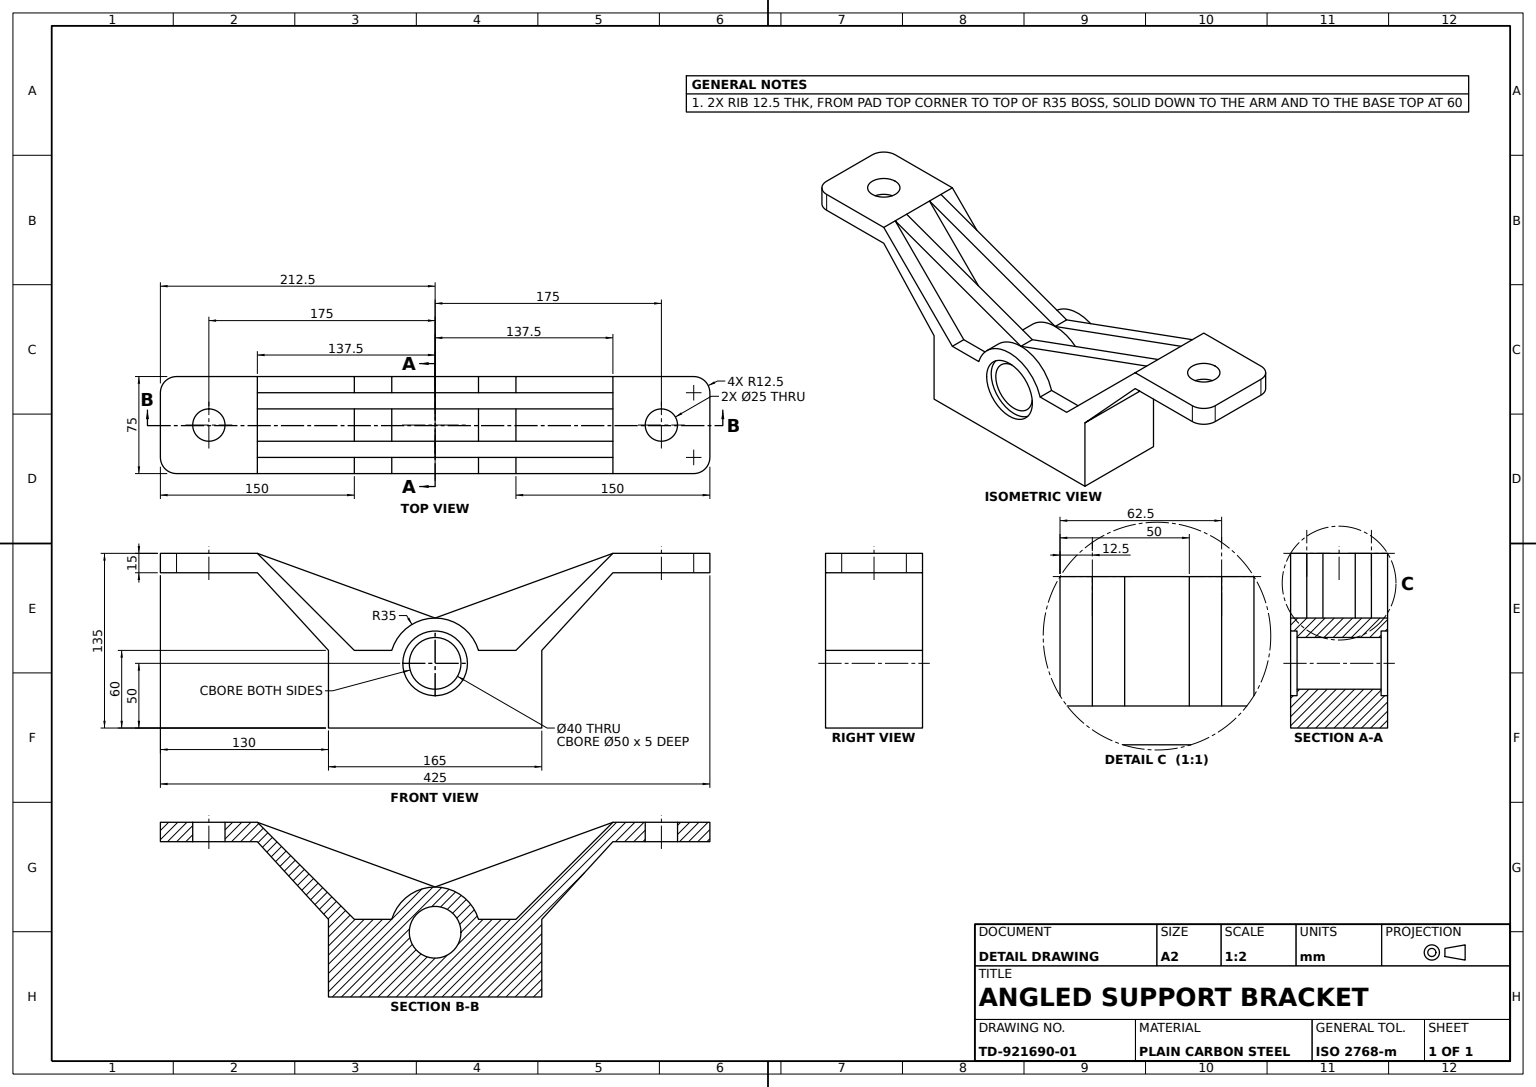
ISO-10303-21;
HEADER;
FILE_DESCRIPTION((''),'2;1');
FILE_NAME('','',(''),(''),'','','');
FILE_SCHEMA(('AUTOMOTIVE_DESIGN'));
ENDSEC;
DATA;
#1=APPLICATION_CONTEXT('');
#2=PRODUCT_CONTEXT('',#1,'mechanical');
#3=PRODUCT('','','',(#2));
#4=PRODUCT_DEFINITION_FORMATION('','',#3);
#5=PRODUCT_DEFINITION_CONTEXT('',#1,'design');
#6=PRODUCT_DEFINITION('','',#4,#5);
#7=PRODUCT_DEFINITION_SHAPE('','',#6);
#8=(LENGTH_UNIT()NAMED_UNIT(*)SI_UNIT(.MILLI.,.METRE.));
#9=(NAMED_UNIT(*)PLANE_ANGLE_UNIT()SI_UNIT($,.RADIAN.));
#10=(NAMED_UNIT(*)SI_UNIT($,.STERADIAN.)SOLID_ANGLE_UNIT());
#11=UNCERTAINTY_MEASURE_WITH_UNIT(LENGTH_MEASURE(1.E-05),#8,'distance_accuracy_value','');
#12=(GEOMETRIC_REPRESENTATION_CONTEXT(3)GLOBAL_UNCERTAINTY_ASSIGNED_CONTEXT((#11))GLOBAL_UNIT_ASSIGNED_CONTEXT((#8,#9,#10))REPRESENTATION_CONTEXT('',''));
#13=CARTESIAN_POINT('',(-212.5,90.,-62.5));
#14=VERTEX_POINT('',#13);
#15=CARTESIAN_POINT('',(-212.5,90.,-12.5));
#16=VERTEX_POINT('',#15);
#17=CARTESIAN_POINT('',(-212.5,90.,-75.));
#18=DIRECTION('',(0.,0.,1.));
#19=VECTOR('',#18,1000.);
#20=LINE('',#17,#19);
#21=EDGE_CURVE('',#14,#16,#20,.T.);
#22=ORIENTED_EDGE('',*,*,#21,.T.);
#23=CARTESIAN_POINT('',(-212.5,105.,-12.5));
#24=VERTEX_POINT('',#23);
#25=CARTESIAN_POINT('',(-212.5,0.,-12.5));
#26=DIRECTION('',(0.,1.,0.));
#27=VECTOR('',#26,1000.);
#28=LINE('',#25,#27);
#29=EDGE_CURVE('',#16,#24,#28,.T.);
#30=ORIENTED_EDGE('',*,*,#29,.T.);
#31=CARTESIAN_POINT('',(-212.5,105.,-62.5));
#32=VERTEX_POINT('',#31);
#33=CARTESIAN_POINT('',(-212.5,105.,-75.));
#34=LINE('',#33,#19);
#35=EDGE_CURVE('',#32,#24,#34,.T.);
#36=ORIENTED_EDGE('',*,*,#35,.F.);
#37=DIRECTION('',(0.,-1.,0.));
#38=VECTOR('',#37,1000.);
#39=LINE('',#13,#38);
#40=EDGE_CURVE('',#32,#14,#39,.T.);
#41=ORIENTED_EDGE('',*,*,#40,.T.);
#42=EDGE_LOOP('',(#22,#30,#36,#41));
#43=FACE_OUTER_BOUND('',#42,.T.);
#44=CARTESIAN_POINT('',(-212.5,0.,-75.));
#45=DIRECTION('',(-1.,0.,0.));
#46=AXIS2_PLACEMENT_3D('',#44,#45,#18);
#47=PLANE('',#46);
#48=ADVANCED_FACE('',(#43),#47,.T.);
#49=CARTESIAN_POINT('',(137.5,105.,-25.));
#50=VERTEX_POINT('',#49);
#51=CARTESIAN_POINT('',(62.5,30.,-25.));
#52=VERTEX_POINT('',#51);
#53=CARTESIAN_POINT('',(16.25,-16.25,-25.));
#54=DIRECTION('',(-0.707106781,-0.707106781,0.));
#55=VECTOR('',#54,1000.);
#56=LINE('',#53,#55);
#57=EDGE_CURVE('',#50,#52,#56,.T.);
#58=ORIENTED_EDGE('',*,*,#57,.F.);
#59=CARTESIAN_POINT('',(137.5,105.,-50.));
#60=VERTEX_POINT('',#59);
#61=CARTESIAN_POINT('',(137.5,105.,-75.));
#62=LINE('',#61,#19);
#63=EDGE_CURVE('',#60,#50,#62,.T.);
#64=ORIENTED_EDGE('',*,*,#63,.F.);
#65=CARTESIAN_POINT('',(62.5,30.,-50.));
#66=VERTEX_POINT('',#65);
#67=CARTESIAN_POINT('',(16.25,-16.25,-50.));
#68=LINE('',#67,#55);
#69=EDGE_CURVE('',#60,#66,#68,.T.);
#70=ORIENTED_EDGE('',*,*,#69,.T.);
#71=CARTESIAN_POINT('',(62.5,30.,-75.));
#72=LINE('',#71,#19);
#73=EDGE_CURVE('',#66,#52,#72,.T.);
#74=ORIENTED_EDGE('',*,*,#73,.T.);
#75=EDGE_LOOP('',(#58,#64,#70,#74));
#76=FACE_OUTER_BOUND('',#75,.T.);
#77=CARTESIAN_POINT('',(16.25,-16.25,-75.));
#78=DIRECTION('',(0.707106781,-0.707106781,0.));
#79=DIRECTION('',(0.707106781,0.707106781,0.));
#80=AXIS2_PLACEMENT_3D('',#77,#78,#79);
#81=PLANE('',#80);
#82=ADVANCED_FACE('',(#76),#81,.F.);
#83=CARTESIAN_POINT('',(-175.,105.,-25.));
#84=VERTEX_POINT('',#83);
#85=CARTESIAN_POINT('',(-175.,105.,-50.));
#86=VERTEX_POINT('',#85);
#87=CARTESIAN_POINT('',(-175.,105.,-37.5));
#88=DIRECTION('',(0.,0.,-1.));
#89=AXIS2_PLACEMENT_3D('',#87,#26,#88);
#90=CIRCLE('',#89,12.5);
#91=EDGE_CURVE('',#84,#86,#90,.T.);
#92=ORIENTED_EDGE('',*,*,#91,.F.);
#93=EDGE_CURVE('',#86,#84,#90,.T.);
#94=ORIENTED_EDGE('',*,*,#93,.F.);
#95=EDGE_LOOP('',(#92,#94));
#96=FACE_BOUND('',#95,.T.);
#97=CARTESIAN_POINT('',(-200.,105.,-75.));
#98=VERTEX_POINT('',#97);
#99=CARTESIAN_POINT('',(-200.,105.,-62.5));
#100=AXIS2_PLACEMENT_3D('',#99,#26,#18);
#101=CIRCLE('',#100,12.5);
#102=EDGE_CURVE('',#98,#32,#101,.T.);
#103=ORIENTED_EDGE('',*,*,#102,.T.);
#104=ORIENTED_EDGE('',*,*,#35,.T.);
#105=CARTESIAN_POINT('',(-200.,105.,0.));
#106=VERTEX_POINT('',#105);
#107=CARTESIAN_POINT('',(-200.,105.,-12.5));
#108=AXIS2_PLACEMENT_3D('',#107,#26,#18);
#109=CIRCLE('',#108,12.5);
#110=EDGE_CURVE('',#24,#106,#109,.T.);
#111=ORIENTED_EDGE('',*,*,#110,.T.);
#112=CARTESIAN_POINT('',(-137.5,105.,0.));
#113=VERTEX_POINT('',#112);
#114=CARTESIAN_POINT('',(0.,105.,0.));
#115=VECTOR('',#45,1000.);
#116=LINE('',#114,#115);
#117=EDGE_CURVE('',#113,#106,#116,.T.);
#118=ORIENTED_EDGE('',*,*,#117,.F.);
#119=CARTESIAN_POINT('',(-137.5,105.,-12.5));
#120=VERTEX_POINT('',#119);
#121=CARTESIAN_POINT('',(-137.5,105.,-75.));
#122=LINE('',#121,#19);
#123=EDGE_CURVE('',#120,#113,#122,.T.);
#124=ORIENTED_EDGE('',*,*,#123,.F.);
#125=CARTESIAN_POINT('',(-137.5,105.,-25.));
#126=VERTEX_POINT('',#125);
#127=LINE('',#125,#19);
#128=EDGE_CURVE('',#126,#120,#127,.T.);
#129=ORIENTED_EDGE('',*,*,#128,.F.);
#130=CARTESIAN_POINT('',(-137.5,105.,-50.));
#131=VERTEX_POINT('',#130);
#132=EDGE_CURVE('',#131,#126,#122,.T.);
#133=ORIENTED_EDGE('',*,*,#132,.F.);
#134=CARTESIAN_POINT('',(-137.5,105.,-62.5));
#135=VERTEX_POINT('',#134);
#136=VECTOR('',#88,1000.);
#137=LINE('',#130,#136);
#138=EDGE_CURVE('',#131,#135,#137,.T.);
#139=ORIENTED_EDGE('',*,*,#138,.T.);
#140=VERTEX_POINT('',#121);
#141=EDGE_CURVE('',#140,#135,#122,.T.);
#142=ORIENTED_EDGE('',*,*,#141,.F.);
#143=CARTESIAN_POINT('',(0.,105.,-75.));
#144=LINE('',#143,#115);
#145=EDGE_CURVE('',#140,#98,#144,.T.);
#146=ORIENTED_EDGE('',*,*,#145,.T.);
#147=EDGE_LOOP('',(#103,#104,#111,#118,#124,#129,#133,#139,#142,#146));
#148=FACE_OUTER_BOUND('',#147,.T.);
#149=AXIS2_PLACEMENT_3D('',#143,#26,#18);
#150=PLANE('',#149);
#151=ADVANCED_FACE('',(#96,#148),#150,.T.);
#152=CARTESIAN_POINT('',(25.,20.,0.));
#153=VERTEX_POINT('',#152);
#154=CARTESIAN_POINT('',(-25.,20.,0.));
#155=VERTEX_POINT('',#154);
#156=CARTESIAN_POINT('',(0.,20.,0.));
#157=DIRECTION('',(1.,0.,0.));
#158=AXIS2_PLACEMENT_3D('',#156,#18,#157);
#159=CIRCLE('',#158,25.);
#160=EDGE_CURVE('',#153,#155,#159,.T.);
#161=ORIENTED_EDGE('',*,*,#160,.F.);
#162=EDGE_CURVE('',#155,#153,#159,.T.);
#163=ORIENTED_EDGE('',*,*,#162,.F.);
#164=EDGE_LOOP('',(#161,#163));
#165=FACE_BOUND('',#164,.T.);
#166=CARTESIAN_POINT('',(-62.5,30.,0.));
#167=VERTEX_POINT('',#166);
#168=CARTESIAN_POINT('',(-16.25,-16.25,0.));
#169=DIRECTION('',(-0.707106781,0.707106781,0.));
#170=VECTOR('',#169,1000.);
#171=LINE('',#168,#170);
#172=EDGE_CURVE('',#167,#113,#171,.T.);
#173=ORIENTED_EDGE('',*,*,#172,.T.);
#174=ORIENTED_EDGE('',*,*,#117,.T.);
#175=CARTESIAN_POINT('',(-200.,90.,0.));
#176=VERTEX_POINT('',#175);
#177=CARTESIAN_POINT('',(-200.,0.,0.));
#178=LINE('',#177,#38);
#179=EDGE_CURVE('',#106,#176,#178,.T.);
#180=ORIENTED_EDGE('',*,*,#179,.T.);
#181=CARTESIAN_POINT('',(-137.5,90.,0.));
#182=VERTEX_POINT('',#181);
#183=CARTESIAN_POINT('',(0.,90.,0.));
#184=VECTOR('',#157,1000.);
#185=LINE('',#183,#184);
#186=EDGE_CURVE('',#176,#182,#185,.T.);
#187=ORIENTED_EDGE('',*,*,#186,.T.);
#188=CARTESIAN_POINT('',(-82.5,30.,0.));
#189=VERTEX_POINT('',#188);
#190=CARTESIAN_POINT('',(-29.886792,-27.396226,0.));
#191=DIRECTION('',(-0.675724629,0.73715414,0.));
#192=VECTOR('',#191,1000.);
#193=LINE('',#190,#192);
#194=EDGE_CURVE('',#189,#182,#193,.T.);
#195=ORIENTED_EDGE('',*,*,#194,.F.);
#196=CARTESIAN_POINT('',(-82.5,-30.,0.));
#197=VERTEX_POINT('',#196);
#198=CARTESIAN_POINT('',(-82.5,0.,0.));
#199=LINE('',#198,#38);
#200=EDGE_CURVE('',#189,#197,#199,.T.);
#201=ORIENTED_EDGE('',*,*,#200,.T.);
#202=CARTESIAN_POINT('',(82.5,-30.,0.));
#203=VERTEX_POINT('',#202);
#204=CARTESIAN_POINT('',(0.,-30.,0.));
#205=LINE('',#204,#184);
#206=EDGE_CURVE('',#197,#203,#205,.T.);
#207=ORIENTED_EDGE('',*,*,#206,.T.);
#208=CARTESIAN_POINT('',(82.5,30.,0.));
#209=VERTEX_POINT('',#208);
#210=CARTESIAN_POINT('',(82.5,0.,0.));
#211=LINE('',#210,#27);
#212=EDGE_CURVE('',#203,#209,#211,.T.);
#213=ORIENTED_EDGE('',*,*,#212,.T.);
#214=CARTESIAN_POINT('',(137.5,90.,0.));
#215=VERTEX_POINT('',#214);
#216=CARTESIAN_POINT('',(29.886792,-27.396226,0.));
#217=DIRECTION('',(0.675724629,0.73715414,0.));
#218=VECTOR('',#217,1000.);
#219=LINE('',#216,#218);
#220=EDGE_CURVE('',#209,#215,#219,.T.);
#221=ORIENTED_EDGE('',*,*,#220,.T.);
#222=CARTESIAN_POINT('',(200.,90.,0.));
#223=VERTEX_POINT('',#222);
#224=LINE('',#183,#115);
#225=EDGE_CURVE('',#223,#215,#224,.T.);
#226=ORIENTED_EDGE('',*,*,#225,.F.);
#227=CARTESIAN_POINT('',(200.,105.,0.));
#228=VERTEX_POINT('',#227);
#229=LINE('',#227,#27);
#230=EDGE_CURVE('',#223,#228,#229,.T.);
#231=ORIENTED_EDGE('',*,*,#230,.T.);
#232=CARTESIAN_POINT('',(137.5,105.,0.));
#233=VERTEX_POINT('',#232);
#234=LINE('',#114,#184);
#235=EDGE_CURVE('',#233,#228,#234,.T.);
#236=ORIENTED_EDGE('',*,*,#235,.F.);
#237=CARTESIAN_POINT('',(62.5,30.,0.));
#238=VERTEX_POINT('',#237);
#239=CARTESIAN_POINT('',(16.25,-16.25,0.));
#240=VECTOR('',#79,1000.);
#241=LINE('',#239,#240);
#242=EDGE_CURVE('',#238,#233,#241,.T.);
#243=ORIENTED_EDGE('',*,*,#242,.F.);
#244=CARTESIAN_POINT('',(33.54102,30.,0.));
#245=VERTEX_POINT('',#244);
#246=CARTESIAN_POINT('',(0.,30.,0.));
#247=LINE('',#246,#184);
#248=EDGE_CURVE('',#245,#238,#247,.T.);
#249=ORIENTED_EDGE('',*,*,#248,.F.);
#250=CARTESIAN_POINT('',(-33.54102,30.,0.));
#251=VERTEX_POINT('',#250);
#252=CIRCLE('',#158,35.);
#253=EDGE_CURVE('',#245,#251,#252,.T.);
#254=ORIENTED_EDGE('',*,*,#253,.T.);
#255=LINE('',#246,#115);
#256=EDGE_CURVE('',#251,#167,#255,.T.);
#257=ORIENTED_EDGE('',*,*,#256,.T.);
#258=EDGE_LOOP('',(#173,#174,#180,#187,#195,#201,#207,#213,#221,#226,#231,#236,#243,#249,#254,#257));
#259=FACE_OUTER_BOUND('',#258,.T.);
#260=CARTESIAN_POINT('',(0.,0.,0.));
#261=AXIS2_PLACEMENT_3D('',#260,#18,#157);
#262=PLANE('',#261);
#263=ADVANCED_FACE('',(#165,#259),#262,.T.);
#264=CARTESIAN_POINT('',(0.,55.,-50.));
#265=VERTEX_POINT('',#264);
#266=CARTESIAN_POINT('',(-17.664234,48.576642,-50.));
#267=DIRECTION('',(0.939793423,0.341743063,0.));
#268=VECTOR('',#267,1000.);
#269=LINE('',#266,#268);
#270=EDGE_CURVE('',#265,#60,#269,.T.);
#271=ORIENTED_EDGE('',*,*,#270,.F.);
#272=CARTESIAN_POINT('',(33.54102,30.,-50.));
#273=VERTEX_POINT('',#272);
#274=CARTESIAN_POINT('',(0.,20.,-50.));
#275=AXIS2_PLACEMENT_3D('',#274,#88,#45);
#276=CIRCLE('',#275,35.);
#277=EDGE_CURVE('',#265,#273,#276,.T.);
#278=ORIENTED_EDGE('',*,*,#277,.T.);
#279=CARTESIAN_POINT('',(0.,30.,-50.));
#280=LINE('',#279,#115);
#281=EDGE_CURVE('',#66,#273,#280,.T.);
#282=ORIENTED_EDGE('',*,*,#281,.F.);
#283=ORIENTED_EDGE('',*,*,#69,.F.);
#284=EDGE_LOOP('',(#271,#278,#282,#283));
#285=FACE_OUTER_BOUND('',#284,.T.);
#286=CARTESIAN_POINT('',(0.,0.,-50.));
#287=AXIS2_PLACEMENT_3D('',#286,#88,#45);
#288=PLANE('',#287);
#289=ADVANCED_FACE('',(#285),#288,.F.);
#290=CARTESIAN_POINT('',(0.,55.,-12.5));
#291=VERTEX_POINT('',#290);
#292=CARTESIAN_POINT('',(17.664234,48.576642,-12.5));
#293=DIRECTION('',(-0.939793423,0.341743063,0.));
#294=VECTOR('',#293,1000.);
#295=LINE('',#292,#294);
#296=EDGE_CURVE('',#291,#120,#295,.T.);
#297=ORIENTED_EDGE('',*,*,#296,.F.);
#298=CARTESIAN_POINT('',(0.,55.,-25.));
#299=VERTEX_POINT('',#298);
#300=LINE('',#298,#19);
#301=EDGE_CURVE('',#299,#291,#300,.T.);
#302=ORIENTED_EDGE('',*,*,#301,.F.);
#303=CARTESIAN_POINT('',(17.664234,48.576642,-25.));
#304=LINE('',#303,#294);
#305=EDGE_CURVE('',#299,#126,#304,.T.);
#306=ORIENTED_EDGE('',*,*,#305,.T.);
#307=ORIENTED_EDGE('',*,*,#128,.T.);
#308=EDGE_LOOP('',(#297,#302,#306,#307));
#309=FACE_OUTER_BOUND('',#308,.T.);
#310=DIRECTION('',(0.341743063,0.939793423,0.));
#311=AXIS2_PLACEMENT_3D('',#303,#310,#293);
#312=PLANE('',#311);
#313=ADVANCED_FACE('',(#309),#312,.T.);
#314=CARTESIAN_POINT('',(200.,90.,-75.));
#315=VERTEX_POINT('',#314);
#316=CARTESIAN_POINT('',(212.5,90.,-62.5));
#317=VERTEX_POINT('',#316);
#318=CARTESIAN_POINT('',(200.,90.,-62.5));
#319=AXIS2_PLACEMENT_3D('',#318,#37,#18);
#320=CIRCLE('',#319,12.5);
#321=EDGE_CURVE('',#315,#317,#320,.T.);
#322=ORIENTED_EDGE('',*,*,#321,.F.);
#323=CARTESIAN_POINT('',(200.,105.,-75.));
#324=VERTEX_POINT('',#323);
#325=CARTESIAN_POINT('',(200.,0.,-75.));
#326=LINE('',#325,#38);
#327=EDGE_CURVE('',#324,#315,#326,.T.);
#328=ORIENTED_EDGE('',*,*,#327,.F.);
#329=CARTESIAN_POINT('',(212.5,105.,-62.5));
#330=VERTEX_POINT('',#329);
#331=CARTESIAN_POINT('',(200.,105.,-62.5));
#332=AXIS2_PLACEMENT_3D('',#331,#26,#88);
#333=CIRCLE('',#332,12.5);
#334=EDGE_CURVE('',#330,#324,#333,.T.);
#335=ORIENTED_EDGE('',*,*,#334,.F.);
#336=CARTESIAN_POINT('',(212.5,0.,-62.5));
#337=LINE('',#336,#27);
#338=EDGE_CURVE('',#317,#330,#337,.T.);
#339=ORIENTED_EDGE('',*,*,#338,.F.);
#340=EDGE_LOOP('',(#322,#328,#335,#339));
#341=FACE_OUTER_BOUND('',#340,.T.);
#342=CARTESIAN_POINT('',(200.,0.,-62.5));
#343=AXIS2_PLACEMENT_3D('',#342,#37,#88);
#344=CYLINDRICAL_SURFACE('',#343,12.5);
#345=ADVANCED_FACE('',(#341),#344,.T.);
#346=CARTESIAN_POINT('',(33.54102,30.,-12.5));
#347=VERTEX_POINT('',#346);
#348=CARTESIAN_POINT('',(33.54102,30.,-75.));
#349=LINE('',#348,#19);
#350=EDGE_CURVE('',#347,#245,#349,.T.);
#351=ORIENTED_EDGE('',*,*,#350,.T.);
#352=ORIENTED_EDGE('',*,*,#248,.T.);
#353=CARTESIAN_POINT('',(62.5,30.,-12.5));
#354=VERTEX_POINT('',#353);
#355=EDGE_CURVE('',#354,#238,#72,.T.);
#356=ORIENTED_EDGE('',*,*,#355,.F.);
#357=CARTESIAN_POINT('',(0.,30.,-12.5));
#358=LINE('',#357,#115);
#359=EDGE_CURVE('',#354,#347,#358,.T.);
#360=ORIENTED_EDGE('',*,*,#359,.T.);
#361=EDGE_LOOP('',(#351,#352,#356,#360));
#362=FACE_OUTER_BOUND('',#361,.T.);
#363=CARTESIAN_POINT('',(0.,30.,-75.));
#364=AXIS2_PLACEMENT_3D('',#363,#37,#157);
#365=PLANE('',#364);
#366=ADVANCED_FACE('',(#362),#365,.F.);
#367=CARTESIAN_POINT('',(212.5,105.,-12.5));
#368=VERTEX_POINT('',#367);
#369=CARTESIAN_POINT('',(212.5,105.,-75.));
#370=LINE('',#369,#19);
#371=EDGE_CURVE('',#330,#368,#370,.T.);
#372=ORIENTED_EDGE('',*,*,#371,.T.);
#373=CARTESIAN_POINT('',(212.5,90.,-12.5));
#374=VERTEX_POINT('',#373);
#375=LINE('',#373,#38);
#376=EDGE_CURVE('',#368,#374,#375,.T.);
#377=ORIENTED_EDGE('',*,*,#376,.T.);
#378=CARTESIAN_POINT('',(212.5,90.,-75.));
#379=LINE('',#378,#19);
#380=EDGE_CURVE('',#317,#374,#379,.T.);
#381=ORIENTED_EDGE('',*,*,#380,.F.);
#382=ORIENTED_EDGE('',*,*,#338,.T.);
#383=EDGE_LOOP('',(#372,#377,#381,#382));
#384=FACE_OUTER_BOUND('',#383,.T.);
#385=CARTESIAN_POINT('',(212.5,0.,-75.));
#386=AXIS2_PLACEMENT_3D('',#385,#45,#18);
#387=PLANE('',#386);
#388=ADVANCED_FACE('',(#384),#387,.F.);
#389=CARTESIAN_POINT('',(-33.54102,30.,-50.));
#390=VERTEX_POINT('',#389);
#391=CARTESIAN_POINT('',(-62.5,30.,-50.));
#392=VERTEX_POINT('',#391);
#393=EDGE_CURVE('',#390,#392,#280,.T.);
#394=ORIENTED_EDGE('',*,*,#393,.T.);
#395=CARTESIAN_POINT('',(-62.5,30.,-25.));
#396=VERTEX_POINT('',#395);
#397=CARTESIAN_POINT('',(-62.5,30.,-75.));
#398=LINE('',#397,#19);
#399=EDGE_CURVE('',#392,#396,#398,.T.);
#400=ORIENTED_EDGE('',*,*,#399,.T.);
#401=CARTESIAN_POINT('',(-33.54102,30.,-25.));
#402=VERTEX_POINT('',#401);
#403=CARTESIAN_POINT('',(0.,30.,-25.));
#404=LINE('',#403,#184);
#405=EDGE_CURVE('',#396,#402,#404,.T.);
#406=ORIENTED_EDGE('',*,*,#405,.T.);
#407=CARTESIAN_POINT('',(-33.54102,30.,-75.));
#408=LINE('',#407,#19);
#409=EDGE_CURVE('',#390,#402,#408,.T.);
#410=ORIENTED_EDGE('',*,*,#409,.F.);
#411=EDGE_LOOP('',(#394,#400,#406,#410));
#412=FACE_OUTER_BOUND('',#411,.T.);
#413=AXIS2_PLACEMENT_3D('',#363,#26,#45);
#414=PLANE('',#413);
#415=ADVANCED_FACE('',(#412),#414,.T.);
#416=CARTESIAN_POINT('',(175.,105.,-50.));
#417=VERTEX_POINT('',#416);
#418=CARTESIAN_POINT('',(175.,105.,-25.));
#419=VERTEX_POINT('',#418);
#420=CARTESIAN_POINT('',(175.,105.,-37.5));
#421=AXIS2_PLACEMENT_3D('',#420,#26,#18);
#422=CIRCLE('',#421,12.5);
#423=EDGE_CURVE('',#417,#419,#422,.T.);
#424=ORIENTED_EDGE('',*,*,#423,.F.);
#425=EDGE_CURVE('',#419,#417,#422,.T.);
#426=ORIENTED_EDGE('',*,*,#425,.F.);
#427=EDGE_LOOP('',(#424,#426));
#428=FACE_BOUND('',#427,.T.);
#429=CARTESIAN_POINT('',(137.5,105.,-62.5));
#430=VERTEX_POINT('',#429);
#431=LINE('',#59,#136);
#432=EDGE_CURVE('',#60,#430,#431,.T.);
#433=ORIENTED_EDGE('',*,*,#432,.F.);
#434=ORIENTED_EDGE('',*,*,#63,.T.);
#435=CARTESIAN_POINT('',(137.5,105.,-12.5));
#436=VERTEX_POINT('',#435);
#437=LINE('',#49,#19);
#438=EDGE_CURVE('',#50,#436,#437,.T.);
#439=ORIENTED_EDGE('',*,*,#438,.T.);
#440=EDGE_CURVE('',#436,#233,#62,.T.);
#441=ORIENTED_EDGE('',*,*,#440,.T.);
#442=ORIENTED_EDGE('',*,*,#235,.T.);
#443=CARTESIAN_POINT('',(200.,105.,-12.5));
#444=AXIS2_PLACEMENT_3D('',#443,#26,#88);
#445=CIRCLE('',#444,12.5);
#446=EDGE_CURVE('',#228,#368,#445,.T.);
#447=ORIENTED_EDGE('',*,*,#446,.T.);
#448=ORIENTED_EDGE('',*,*,#371,.F.);
#449=ORIENTED_EDGE('',*,*,#334,.T.);
#450=VERTEX_POINT('',#61);
#451=LINE('',#143,#184);
#452=EDGE_CURVE('',#450,#324,#451,.T.);
#453=ORIENTED_EDGE('',*,*,#452,.F.);
#454=EDGE_CURVE('',#450,#430,#62,.T.);
#455=ORIENTED_EDGE('',*,*,#454,.T.);
#456=EDGE_LOOP('',(#433,#434,#439,#441,#442,#447,#448,#449,#453,#455));
#457=FACE_OUTER_BOUND('',#456,.T.);
#458=AXIS2_PLACEMENT_3D('',#143,#37,#88);
#459=PLANE('',#458);
#460=ADVANCED_FACE('',(#428,#457),#459,.F.);
#461=CARTESIAN_POINT('',(25.,20.,-5.));
#462=VERTEX_POINT('',#461);
#463=LINE('',#461,#19);
#464=EDGE_CURVE('',#462,#153,#463,.T.);
#465=ORIENTED_EDGE('',*,*,#464,.T.);
#466=ORIENTED_EDGE('',*,*,#160,.T.);
#467=CARTESIAN_POINT('',(-25.,20.,-5.));
#468=VERTEX_POINT('',#467);
#469=LINE('',#467,#19);
#470=EDGE_CURVE('',#468,#155,#469,.T.);
#471=ORIENTED_EDGE('',*,*,#470,.F.);
#472=CARTESIAN_POINT('',(0.,20.,-5.));
#473=AXIS2_PLACEMENT_3D('',#472,#18,#157);
#474=CIRCLE('',#473,25.);
#475=EDGE_CURVE('',#462,#468,#474,.T.);
#476=ORIENTED_EDGE('',*,*,#475,.F.);
#477=EDGE_LOOP('',(#465,#466,#471,#476));
#478=FACE_OUTER_BOUND('',#477,.T.);
#479=CYLINDRICAL_SURFACE('',#473,25.);
#480=ADVANCED_FACE('',(#478),#479,.F.);
#481=CARTESIAN_POINT('',(82.5,30.,-75.));
#482=VERTEX_POINT('',#481);
#483=CARTESIAN_POINT('',(137.5,90.,-75.));
#484=VERTEX_POINT('',#483);
#485=CARTESIAN_POINT('',(29.886792,-27.396226,-75.));
#486=LINE('',#485,#218);
#487=EDGE_CURVE('',#482,#484,#486,.T.);
#488=ORIENTED_EDGE('',*,*,#487,.T.);
#489=LINE('',#483,#19);
#490=EDGE_CURVE('',#484,#215,#489,.T.);
#491=ORIENTED_EDGE('',*,*,#490,.T.);
#492=ORIENTED_EDGE('',*,*,#220,.F.);
#493=LINE('',#481,#19);
#494=EDGE_CURVE('',#482,#209,#493,.T.);
#495=ORIENTED_EDGE('',*,*,#494,.F.);
#496=EDGE_LOOP('',(#488,#491,#492,#495));
#497=FACE_OUTER_BOUND('',#496,.T.);
#498=DIRECTION('',(0.73715414,-0.675724629,0.));
#499=AXIS2_PLACEMENT_3D('',#485,#498,#217);
#500=PLANE('',#499);
#501=ADVANCED_FACE('',(#497),#500,.T.);
#502=CARTESIAN_POINT('',(0.,20.,-25.));
#503=AXIS2_PLACEMENT_3D('',#502,#18,#157);
#504=CIRCLE('',#503,35.);
#505=EDGE_CURVE('',#299,#402,#504,.T.);
#506=ORIENTED_EDGE('',*,*,#505,.T.);
#507=ORIENTED_EDGE('',*,*,#405,.F.);
#508=CARTESIAN_POINT('',(-16.25,-16.25,-25.));
#509=VECTOR('',#78,1000.);
#510=LINE('',#508,#509);
#511=EDGE_CURVE('',#126,#396,#510,.T.);
#512=ORIENTED_EDGE('',*,*,#511,.F.);
#513=ORIENTED_EDGE('',*,*,#305,.F.);
#514=EDGE_LOOP('',(#506,#507,#512,#513));
#515=FACE_OUTER_BOUND('',#514,.T.);
#516=CARTESIAN_POINT('',(0.,0.,-25.));
#517=AXIS2_PLACEMENT_3D('',#516,#18,#157);
#518=PLANE('',#517);
#519=ADVANCED_FACE('',(#515),#518,.F.);
#520=CARTESIAN_POINT('',(-175.,90.,-50.));
#521=VERTEX_POINT('',#520);
#522=CARTESIAN_POINT('',(-175.,-3.5,-50.));
#523=LINE('',#522,#27);
#524=EDGE_CURVE('',#521,#86,#523,.T.);
#525=ORIENTED_EDGE('',*,*,#524,.F.);
#526=CARTESIAN_POINT('',(-175.,90.,-25.));
#527=VERTEX_POINT('',#526);
#528=CARTESIAN_POINT('',(-175.,90.,-37.5));
#529=AXIS2_PLACEMENT_3D('',#528,#37,#88);
#530=CIRCLE('',#529,12.5);
#531=EDGE_CURVE('',#521,#527,#530,.T.);
#532=ORIENTED_EDGE('',*,*,#531,.T.);
#533=CARTESIAN_POINT('',(-175.,-3.5,-25.));
#534=LINE('',#533,#27);
#535=EDGE_CURVE('',#527,#84,#534,.T.);
#536=ORIENTED_EDGE('',*,*,#535,.T.);
#537=ORIENTED_EDGE('',*,*,#91,.T.);
#538=EDGE_LOOP('',(#525,#532,#536,#537));
#539=FACE_OUTER_BOUND('',#538,.T.);
#540=CARTESIAN_POINT('',(-175.,-3.5,-37.5));
#541=AXIS2_PLACEMENT_3D('',#540,#26,#18);
#542=CYLINDRICAL_SURFACE('',#541,12.5);
#543=ADVANCED_FACE('',(#539),#542,.F.);
#544=CARTESIAN_POINT('',(0.,20.,-12.5));
#545=AXIS2_PLACEMENT_3D('',#544,#18,#157);
#546=CIRCLE('',#545,35.);
#547=EDGE_CURVE('',#347,#291,#546,.T.);
#548=ORIENTED_EDGE('',*,*,#547,.F.);
#549=ORIENTED_EDGE('',*,*,#359,.F.);
#550=CARTESIAN_POINT('',(16.25,-16.25,-12.5));
#551=LINE('',#550,#55);
#552=EDGE_CURVE('',#436,#354,#551,.T.);
#553=ORIENTED_EDGE('',*,*,#552,.F.);
#554=CARTESIAN_POINT('',(-17.664234,48.576642,-12.5));
#555=LINE('',#554,#268);
#556=EDGE_CURVE('',#291,#436,#555,.T.);
#557=ORIENTED_EDGE('',*,*,#556,.F.);
#558=EDGE_LOOP('',(#548,#549,#553,#557));
#559=FACE_OUTER_BOUND('',#558,.T.);
#560=CARTESIAN_POINT('',(0.,0.,-12.5));
#561=AXIS2_PLACEMENT_3D('',#560,#18,#157);
#562=PLANE('',#561);
#563=ADVANCED_FACE('',(#559),#562,.T.);
#564=ORIENTED_EDGE('',*,*,#475,.T.);
#565=EDGE_CURVE('',#468,#462,#474,.T.);
#566=ORIENTED_EDGE('',*,*,#565,.T.);
#567=EDGE_LOOP('',(#564,#566));
#568=FACE_OUTER_BOUND('',#567,.T.);
#569=CARTESIAN_POINT('',(20.,20.,-5.));
#570=VERTEX_POINT('',#569);
#571=CARTESIAN_POINT('',(-20.,20.,-5.));
#572=VERTEX_POINT('',#571);
#573=CIRCLE('',#473,20.);
#574=EDGE_CURVE('',#570,#572,#573,.T.);
#575=ORIENTED_EDGE('',*,*,#574,.F.);
#576=EDGE_CURVE('',#572,#570,#573,.T.);
#577=ORIENTED_EDGE('',*,*,#576,.F.);
#578=EDGE_LOOP('',(#575,#577));
#579=FACE_BOUND('',#578,.T.);
#580=PLANE('',#473);
#581=ADVANCED_FACE('',(#568,#579),#580,.T.);
#582=ORIENTED_EDGE('',*,*,#565,.F.);
#583=ORIENTED_EDGE('',*,*,#470,.T.);
#584=ORIENTED_EDGE('',*,*,#162,.T.);
#585=ORIENTED_EDGE('',*,*,#464,.F.);
#586=EDGE_LOOP('',(#582,#583,#584,#585));
#587=FACE_OUTER_BOUND('',#586,.T.);
#588=ADVANCED_FACE('',(#587),#479,.F.);
#589=CARTESIAN_POINT('',(-17.664234,48.576642,-25.));
#590=LINE('',#589,#268);
#591=EDGE_CURVE('',#299,#50,#590,.T.);
#592=ORIENTED_EDGE('',*,*,#591,.F.);
#593=ORIENTED_EDGE('',*,*,#301,.T.);
#594=ORIENTED_EDGE('',*,*,#556,.T.);
#595=ORIENTED_EDGE('',*,*,#438,.F.);
#596=EDGE_LOOP('',(#592,#593,#594,#595));
#597=FACE_OUTER_BOUND('',#596,.T.);
#598=DIRECTION('',(0.341743063,-0.939793423,0.));
#599=AXIS2_PLACEMENT_3D('',#589,#598,#267);
#600=PLANE('',#599);
#601=ADVANCED_FACE('',(#597),#600,.F.);
#602=CARTESIAN_POINT('',(0.,90.,-75.));
#603=LINE('',#602,#115);
#604=EDGE_CURVE('',#315,#484,#603,.T.);
#605=ORIENTED_EDGE('',*,*,#604,.F.);
#606=ORIENTED_EDGE('',*,*,#321,.T.);
#607=ORIENTED_EDGE('',*,*,#380,.T.);
#608=CARTESIAN_POINT('',(200.,90.,-12.5));
#609=AXIS2_PLACEMENT_3D('',#608,#37,#18);
#610=CIRCLE('',#609,12.5);
#611=EDGE_CURVE('',#374,#223,#610,.T.);
#612=ORIENTED_EDGE('',*,*,#611,.T.);
#613=ORIENTED_EDGE('',*,*,#225,.T.);
#614=ORIENTED_EDGE('',*,*,#490,.F.);
#615=EDGE_LOOP('',(#605,#606,#607,#612,#613,#614));
#616=FACE_OUTER_BOUND('',#615,.T.);
#617=CARTESIAN_POINT('',(175.,90.,-50.));
#618=VERTEX_POINT('',#617);
#619=CARTESIAN_POINT('',(175.,90.,-25.));
#620=VERTEX_POINT('',#619);
#621=CARTESIAN_POINT('',(175.,90.,-37.5));
#622=AXIS2_PLACEMENT_3D('',#621,#26,#18);
#623=CIRCLE('',#622,12.5);
#624=EDGE_CURVE('',#618,#620,#623,.T.);
#625=ORIENTED_EDGE('',*,*,#624,.T.);
#626=EDGE_CURVE('',#620,#618,#623,.T.);
#627=ORIENTED_EDGE('',*,*,#626,.T.);
#628=EDGE_LOOP('',(#625,#627));
#629=FACE_BOUND('',#628,.T.);
#630=AXIS2_PLACEMENT_3D('',#602,#26,#18);
#631=PLANE('',#630);
#632=ADVANCED_FACE('',(#616,#629),#631,.F.);
#633=CARTESIAN_POINT('',(0.,55.,-62.5));
#634=VERTEX_POINT('',#633);
#635=CARTESIAN_POINT('',(-17.664234,48.576642,-62.5));
#636=LINE('',#635,#268);
#637=EDGE_CURVE('',#634,#430,#636,.T.);
#638=ORIENTED_EDGE('',*,*,#637,.T.);
#639=CARTESIAN_POINT('',(62.5,30.,-62.5));
#640=VERTEX_POINT('',#639);
#641=CARTESIAN_POINT('',(16.25,-16.25,-62.5));
#642=LINE('',#641,#55);
#643=EDGE_CURVE('',#430,#640,#642,.T.);
#644=ORIENTED_EDGE('',*,*,#643,.T.);
#645=CARTESIAN_POINT('',(33.54102,30.,-62.5));
#646=VERTEX_POINT('',#645);
#647=CARTESIAN_POINT('',(0.,30.,-62.5));
#648=LINE('',#647,#115);
#649=EDGE_CURVE('',#640,#646,#648,.T.);
#650=ORIENTED_EDGE('',*,*,#649,.T.);
#651=CARTESIAN_POINT('',(0.,20.,-62.5));
#652=AXIS2_PLACEMENT_3D('',#651,#88,#45);
#653=CIRCLE('',#652,35.);
#654=EDGE_CURVE('',#634,#646,#653,.T.);
#655=ORIENTED_EDGE('',*,*,#654,.F.);
#656=EDGE_LOOP('',(#638,#644,#650,#655));
#657=FACE_OUTER_BOUND('',#656,.T.);
#658=CARTESIAN_POINT('',(0.,0.,-62.5));
#659=AXIS2_PLACEMENT_3D('',#658,#88,#45);
#660=PLANE('',#659);
#661=ADVANCED_FACE('',(#657),#660,.T.);
#662=ORIENTED_EDGE('',*,*,#649,.F.);
#663=VERTEX_POINT('',#71);
#664=EDGE_CURVE('',#663,#640,#72,.T.);
#665=ORIENTED_EDGE('',*,*,#664,.F.);
#666=VERTEX_POINT('',#348);
#667=LINE('',#363,#184);
#668=EDGE_CURVE('',#666,#663,#667,.T.);
#669=ORIENTED_EDGE('',*,*,#668,.F.);
#670=EDGE_CURVE('',#666,#646,#349,.T.);
#671=ORIENTED_EDGE('',*,*,#670,.T.);
#672=EDGE_LOOP('',(#662,#665,#669,#671));
#673=FACE_OUTER_BOUND('',#672,.T.);
#674=ADVANCED_FACE('',(#673),#365,.F.);
#675=LINE('',#264,#136);
#676=EDGE_CURVE('',#265,#634,#675,.T.);
#677=ORIENTED_EDGE('',*,*,#676,.T.);
#678=CARTESIAN_POINT('',(17.664234,48.576642,-62.5));
#679=DIRECTION('',(0.939793423,-0.341743063,0.));
#680=VECTOR('',#679,1000.);
#681=LINE('',#678,#680);
#682=EDGE_CURVE('',#135,#634,#681,.T.);
#683=ORIENTED_EDGE('',*,*,#682,.F.);
#684=ORIENTED_EDGE('',*,*,#138,.F.);
#685=CARTESIAN_POINT('',(17.664234,48.576642,-50.));
#686=LINE('',#685,#680);
#687=EDGE_CURVE('',#131,#265,#686,.T.);
#688=ORIENTED_EDGE('',*,*,#687,.T.);
#689=EDGE_LOOP('',(#677,#683,#684,#688));
#690=FACE_OUTER_BOUND('',#689,.T.);
#691=AXIS2_PLACEMENT_3D('',#685,#310,#293);
#692=PLANE('',#691);
#693=ADVANCED_FACE('',(#690),#692,.T.);
#694=ORIENTED_EDGE('',*,*,#687,.F.);
#695=CARTESIAN_POINT('',(-16.25,-16.25,-50.));
#696=LINE('',#695,#170);
#697=EDGE_CURVE('',#392,#131,#696,.T.);
#698=ORIENTED_EDGE('',*,*,#697,.F.);
#699=ORIENTED_EDGE('',*,*,#393,.F.);
#700=EDGE_CURVE('',#390,#265,#276,.T.);
#701=ORIENTED_EDGE('',*,*,#700,.T.);
#702=EDGE_LOOP('',(#694,#698,#699,#701));
#703=FACE_OUTER_BOUND('',#702,.T.);
#704=ADVANCED_FACE('',(#703),#288,.F.);
#705=CARTESIAN_POINT('',(33.54102,30.,-25.));
#706=VERTEX_POINT('',#705);
#707=LINE('',#403,#115);
#708=EDGE_CURVE('',#52,#706,#707,.T.);
#709=ORIENTED_EDGE('',*,*,#708,.T.);
#710=EDGE_CURVE('',#706,#299,#504,.T.);
#711=ORIENTED_EDGE('',*,*,#710,.T.);
#712=ORIENTED_EDGE('',*,*,#591,.T.);
#713=ORIENTED_EDGE('',*,*,#57,.T.);
#714=EDGE_LOOP('',(#709,#711,#712,#713));
#715=FACE_OUTER_BOUND('',#714,.T.);
#716=ADVANCED_FACE('',(#715),#518,.F.);
#717=ORIENTED_EDGE('',*,*,#531,.F.);
#718=EDGE_CURVE('',#527,#521,#530,.T.);
#719=ORIENTED_EDGE('',*,*,#718,.F.);
#720=EDGE_LOOP('',(#717,#719));
#721=FACE_BOUND('',#720,.T.);
#722=ORIENTED_EDGE('',*,*,#186,.F.);
#723=CARTESIAN_POINT('',(-200.,90.,-12.5));
#724=AXIS2_PLACEMENT_3D('',#723,#37,#88);
#725=CIRCLE('',#724,12.5);
#726=EDGE_CURVE('',#176,#16,#725,.T.);
#727=ORIENTED_EDGE('',*,*,#726,.T.);
#728=ORIENTED_EDGE('',*,*,#21,.F.);
#729=CARTESIAN_POINT('',(-200.,90.,-75.));
#730=VERTEX_POINT('',#729);
#731=CARTESIAN_POINT('',(-200.,90.,-62.5));
#732=AXIS2_PLACEMENT_3D('',#731,#37,#88);
#733=CIRCLE('',#732,12.5);
#734=EDGE_CURVE('',#14,#730,#733,.T.);
#735=ORIENTED_EDGE('',*,*,#734,.T.);
#736=CARTESIAN_POINT('',(-137.5,90.,-75.));
#737=VERTEX_POINT('',#736);
#738=LINE('',#602,#184);
#739=EDGE_CURVE('',#730,#737,#738,.T.);
#740=ORIENTED_EDGE('',*,*,#739,.T.);
#741=LINE('',#736,#19);
#742=EDGE_CURVE('',#737,#182,#741,.T.);
#743=ORIENTED_EDGE('',*,*,#742,.T.);
#744=EDGE_LOOP('',(#722,#727,#728,#735,#740,#743));
#745=FACE_OUTER_BOUND('',#744,.T.);
#746=AXIS2_PLACEMENT_3D('',#602,#37,#88);
#747=PLANE('',#746);
#748=ADVANCED_FACE('',(#721,#745),#747,.T.);
#749=ORIENTED_EDGE('',*,*,#708,.F.);
#750=ORIENTED_EDGE('',*,*,#73,.F.);
#751=ORIENTED_EDGE('',*,*,#281,.T.);
#752=EDGE_CURVE('',#273,#706,#349,.T.);
#753=ORIENTED_EDGE('',*,*,#752,.T.);
#754=EDGE_LOOP('',(#749,#750,#751,#753));
#755=FACE_OUTER_BOUND('',#754,.T.);
#756=ADVANCED_FACE('',(#755),#365,.F.);
#757=VERTEX_POINT('',#407);
#758=CARTESIAN_POINT('',(-33.54102,30.,-62.5));
#759=VERTEX_POINT('',#758);
#760=EDGE_CURVE('',#757,#759,#408,.T.);
#761=ORIENTED_EDGE('',*,*,#760,.F.);
#762=VERTEX_POINT('',#397);
#763=LINE('',#363,#115);
#764=EDGE_CURVE('',#757,#762,#763,.T.);
#765=ORIENTED_EDGE('',*,*,#764,.T.);
#766=CARTESIAN_POINT('',(-62.5,30.,-62.5));
#767=VERTEX_POINT('',#766);
#768=EDGE_CURVE('',#762,#767,#398,.T.);
#769=ORIENTED_EDGE('',*,*,#768,.T.);
#770=EDGE_CURVE('',#759,#767,#648,.T.);
#771=ORIENTED_EDGE('',*,*,#770,.F.);
#772=EDGE_LOOP('',(#761,#765,#769,#771));
#773=FACE_OUTER_BOUND('',#772,.T.);
#774=ADVANCED_FACE('',(#773),#414,.T.);
#775=ORIENTED_EDGE('',*,*,#206,.F.);
#776=CARTESIAN_POINT('',(-82.5,-30.,-75.));
#777=VERTEX_POINT('',#776);
#778=LINE('',#776,#19);
#779=EDGE_CURVE('',#777,#197,#778,.T.);
#780=ORIENTED_EDGE('',*,*,#779,.F.);
#781=CARTESIAN_POINT('',(82.5,-30.,-75.));
#782=VERTEX_POINT('',#781);
#783=CARTESIAN_POINT('',(0.,-30.,-75.));
#784=LINE('',#783,#184);
#785=EDGE_CURVE('',#777,#782,#784,.T.);
#786=ORIENTED_EDGE('',*,*,#785,.T.);
#787=LINE('',#781,#19);
#788=EDGE_CURVE('',#782,#203,#787,.T.);
#789=ORIENTED_EDGE('',*,*,#788,.T.);
#790=EDGE_LOOP('',(#775,#780,#786,#789));
#791=FACE_OUTER_BOUND('',#790,.T.);
#792=AXIS2_PLACEMENT_3D('',#783,#37,#88);
#793=PLANE('',#792);
#794=ADVANCED_FACE('',(#791),#793,.T.);
#795=CARTESIAN_POINT('',(-62.5,30.,-12.5));
#796=VERTEX_POINT('',#795);
#797=EDGE_CURVE('',#796,#167,#398,.T.);
#798=ORIENTED_EDGE('',*,*,#797,.F.);
#799=CARTESIAN_POINT('',(-16.25,-16.25,-12.5));
#800=LINE('',#799,#509);
#801=EDGE_CURVE('',#120,#796,#800,.T.);
#802=ORIENTED_EDGE('',*,*,#801,.F.);
#803=ORIENTED_EDGE('',*,*,#123,.T.);
#804=ORIENTED_EDGE('',*,*,#172,.F.);
#805=EDGE_LOOP('',(#798,#802,#803,#804));
#806=FACE_OUTER_BOUND('',#805,.T.);
#807=CARTESIAN_POINT('',(-16.25,-16.25,-75.));
#808=AXIS2_PLACEMENT_3D('',#807,#79,#169);
#809=PLANE('',#808);
#810=ADVANCED_FACE('',(#806),#809,.T.);
#811=ORIENTED_EDGE('',*,*,#454,.F.);
#812=LINE('',#77,#240);
#813=EDGE_CURVE('',#663,#450,#812,.T.);
#814=ORIENTED_EDGE('',*,*,#813,.F.);
#815=ORIENTED_EDGE('',*,*,#664,.T.);
#816=ORIENTED_EDGE('',*,*,#643,.F.);
#817=EDGE_LOOP('',(#811,#814,#815,#816));
#818=FACE_OUTER_BOUND('',#817,.T.);
#819=ADVANCED_FACE('',(#818),#81,.F.);
#820=ORIENTED_EDGE('',*,*,#574,.T.);
#821=CARTESIAN_POINT('',(-20.,20.,-70.));
#822=VERTEX_POINT('',#821);
#823=CARTESIAN_POINT('',(-20.,20.,-103.));
#824=LINE('',#823,#19);
#825=EDGE_CURVE('',#822,#572,#824,.T.);
#826=ORIENTED_EDGE('',*,*,#825,.F.);
#827=CARTESIAN_POINT('',(20.,20.,-70.));
#828=VERTEX_POINT('',#827);
#829=CARTESIAN_POINT('',(0.,20.,-70.));
#830=AXIS2_PLACEMENT_3D('',#829,#18,#45);
#831=CIRCLE('',#830,20.);
#832=EDGE_CURVE('',#828,#822,#831,.T.);
#833=ORIENTED_EDGE('',*,*,#832,.F.);
#834=CARTESIAN_POINT('',(20.,20.,-103.));
#835=LINE('',#834,#19);
#836=EDGE_CURVE('',#828,#570,#835,.T.);
#837=ORIENTED_EDGE('',*,*,#836,.T.);
#838=EDGE_LOOP('',(#820,#826,#833,#837));
#839=FACE_OUTER_BOUND('',#838,.T.);
#840=CARTESIAN_POINT('',(0.,20.,-103.));
#841=AXIS2_PLACEMENT_3D('',#840,#18,#157);
#842=CYLINDRICAL_SURFACE('',#841,20.);
#843=ADVANCED_FACE('',(#839),#842,.F.);
#844=ORIENTED_EDGE('',*,*,#832,.T.);
#845=EDGE_CURVE('',#822,#828,#831,.T.);
#846=ORIENTED_EDGE('',*,*,#845,.T.);
#847=EDGE_LOOP('',(#844,#846));
#848=FACE_BOUND('',#847,.T.);
#849=CARTESIAN_POINT('',(-25.,20.,-70.));
#850=VERTEX_POINT('',#849);
#851=CARTESIAN_POINT('',(25.,20.,-70.));
#852=VERTEX_POINT('',#851);
#853=AXIS2_PLACEMENT_3D('',#829,#88,#45);
#854=CIRCLE('',#853,25.);
#855=EDGE_CURVE('',#850,#852,#854,.T.);
#856=ORIENTED_EDGE('',*,*,#855,.T.);
#857=EDGE_CURVE('',#852,#850,#854,.T.);
#858=ORIENTED_EDGE('',*,*,#857,.T.);
#859=EDGE_LOOP('',(#856,#858));
#860=FACE_OUTER_BOUND('',#859,.T.);
#861=PLANE('',#853);
#862=ADVANCED_FACE('',(#848,#860),#861,.T.);
#863=ORIENTED_EDGE('',*,*,#425,.T.);
#864=CARTESIAN_POINT('',(175.,-3.5,-50.));
#865=LINE('',#864,#27);
#866=EDGE_CURVE('',#618,#417,#865,.T.);
#867=ORIENTED_EDGE('',*,*,#866,.F.);
#868=ORIENTED_EDGE('',*,*,#626,.F.);
#869=CARTESIAN_POINT('',(175.,-3.5,-25.));
#870=LINE('',#869,#27);
#871=EDGE_CURVE('',#620,#419,#870,.T.);
#872=ORIENTED_EDGE('',*,*,#871,.T.);
#873=EDGE_LOOP('',(#863,#867,#868,#872));
#874=FACE_OUTER_BOUND('',#873,.T.);
#875=CARTESIAN_POINT('',(175.,-3.5,-37.5));
#876=AXIS2_PLACEMENT_3D('',#875,#26,#18);
#877=CYLINDRICAL_SURFACE('',#876,12.5);
#878=ADVANCED_FACE('',(#874),#877,.F.);
#879=ORIENTED_EDGE('',*,*,#494,.T.);
#880=ORIENTED_EDGE('',*,*,#212,.F.);
#881=ORIENTED_EDGE('',*,*,#788,.F.);
#882=CARTESIAN_POINT('',(82.5,0.,-75.));
#883=LINE('',#882,#27);
#884=EDGE_CURVE('',#782,#482,#883,.T.);
#885=ORIENTED_EDGE('',*,*,#884,.T.);
#886=EDGE_LOOP('',(#879,#880,#881,#885));
#887=FACE_OUTER_BOUND('',#886,.T.);
#888=AXIS2_PLACEMENT_3D('',#882,#157,#88);
#889=PLANE('',#888);
#890=ADVANCED_FACE('',(#887),#889,.T.);
#891=ORIENTED_EDGE('',*,*,#855,.F.);
#892=CARTESIAN_POINT('',(-25.,20.,-75.));
#893=VERTEX_POINT('',#892);
#894=LINE('',#849,#136);
#895=EDGE_CURVE('',#850,#893,#894,.T.);
#896=ORIENTED_EDGE('',*,*,#895,.T.);
#897=CARTESIAN_POINT('',(25.,20.,-75.));
#898=VERTEX_POINT('',#897);
#899=CARTESIAN_POINT('',(0.,20.,-75.));
#900=AXIS2_PLACEMENT_3D('',#899,#88,#45);
#901=CIRCLE('',#900,25.);
#902=EDGE_CURVE('',#893,#898,#901,.T.);
#903=ORIENTED_EDGE('',*,*,#902,.T.);
#904=LINE('',#851,#136);
#905=EDGE_CURVE('',#852,#898,#904,.T.);
#906=ORIENTED_EDGE('',*,*,#905,.F.);
#907=EDGE_LOOP('',(#891,#896,#903,#906));
#908=FACE_OUTER_BOUND('',#907,.T.);
#909=CYLINDRICAL_SURFACE('',#853,25.);
#910=ADVANCED_FACE('',(#908),#909,.F.);
#911=ORIENTED_EDGE('',*,*,#432,.T.);
#912=ORIENTED_EDGE('',*,*,#637,.F.);
#913=ORIENTED_EDGE('',*,*,#676,.F.);
#914=ORIENTED_EDGE('',*,*,#270,.T.);
#915=EDGE_LOOP('',(#911,#912,#913,#914));
#916=FACE_OUTER_BOUND('',#915,.T.);
#917=DIRECTION('',(-0.341743063,0.939793423,0.));
#918=DIRECTION('',(-0.939793423,-0.341743063,0.));
#919=AXIS2_PLACEMENT_3D('',#266,#917,#918);
#920=PLANE('',#919);
#921=ADVANCED_FACE('',(#916),#920,.T.);
#922=ORIENTED_EDGE('',*,*,#256,.F.);
#923=CARTESIAN_POINT('',(-33.54102,30.,-12.5));
#924=VERTEX_POINT('',#923);
#925=EDGE_CURVE('',#924,#251,#408,.T.);
#926=ORIENTED_EDGE('',*,*,#925,.F.);
#927=LINE('',#357,#184);
#928=EDGE_CURVE('',#796,#924,#927,.T.);
#929=ORIENTED_EDGE('',*,*,#928,.F.);
#930=ORIENTED_EDGE('',*,*,#797,.T.);
#931=EDGE_LOOP('',(#922,#926,#929,#930));
#932=FACE_OUTER_BOUND('',#931,.T.);
#933=ADVANCED_FACE('',(#932),#414,.T.);
#934=LINE('',#807,#170);
#935=EDGE_CURVE('',#762,#140,#934,.T.);
#936=ORIENTED_EDGE('',*,*,#935,.T.);
#937=ORIENTED_EDGE('',*,*,#141,.T.);
#938=CARTESIAN_POINT('',(-16.25,-16.25,-62.5));
#939=LINE('',#938,#170);
#940=EDGE_CURVE('',#767,#135,#939,.T.);
#941=ORIENTED_EDGE('',*,*,#940,.F.);
#942=ORIENTED_EDGE('',*,*,#768,.F.);
#943=EDGE_LOOP('',(#936,#937,#941,#942));
#944=FACE_OUTER_BOUND('',#943,.T.);
#945=ADVANCED_FACE('',(#944),#809,.T.);
#946=ORIENTED_EDGE('',*,*,#505,.F.);
#947=ORIENTED_EDGE('',*,*,#710,.F.);
#948=ORIENTED_EDGE('',*,*,#752,.F.);
#949=ORIENTED_EDGE('',*,*,#277,.F.);
#950=ORIENTED_EDGE('',*,*,#700,.F.);
#951=ORIENTED_EDGE('',*,*,#409,.T.);
#952=EDGE_LOOP('',(#946,#947,#948,#949,#950,#951));
#953=FACE_OUTER_BOUND('',#952,.T.);
#954=AXIS2_PLACEMENT_3D('',#899,#18,#157);
#955=CYLINDRICAL_SURFACE('',#954,35.);
#956=ADVANCED_FACE('',(#953),#955,.T.);
#957=ORIENTED_EDGE('',*,*,#132,.T.);
#958=ORIENTED_EDGE('',*,*,#511,.T.);
#959=ORIENTED_EDGE('',*,*,#399,.F.);
#960=ORIENTED_EDGE('',*,*,#697,.T.);
#961=EDGE_LOOP('',(#957,#958,#959,#960));
#962=FACE_OUTER_BOUND('',#961,.T.);
#963=ADVANCED_FACE('',(#962),#809,.T.);
#964=ORIENTED_EDGE('',*,*,#40,.F.);
#965=ORIENTED_EDGE('',*,*,#102,.F.);
#966=LINE('',#97,#27);
#967=EDGE_CURVE('',#730,#98,#966,.T.);
#968=ORIENTED_EDGE('',*,*,#967,.F.);
#969=ORIENTED_EDGE('',*,*,#734,.F.);
#970=EDGE_LOOP('',(#964,#965,#968,#969));
#971=FACE_OUTER_BOUND('',#970,.T.);
#972=CARTESIAN_POINT('',(-200.,0.,-62.5));
#973=AXIS2_PLACEMENT_3D('',#972,#26,#18);
#974=CYLINDRICAL_SURFACE('',#973,12.5);
#975=ADVANCED_FACE('',(#971),#974,.T.);
#976=EDGE_CURVE('',#759,#634,#653,.T.);
#977=ORIENTED_EDGE('',*,*,#976,.F.);
#978=ORIENTED_EDGE('',*,*,#770,.T.);
#979=ORIENTED_EDGE('',*,*,#940,.T.);
#980=ORIENTED_EDGE('',*,*,#682,.T.);
#981=EDGE_LOOP('',(#977,#978,#979,#980));
#982=FACE_OUTER_BOUND('',#981,.T.);
#983=ADVANCED_FACE('',(#982),#660,.T.);
#984=ORIENTED_EDGE('',*,*,#857,.F.);
#985=ORIENTED_EDGE('',*,*,#905,.T.);
#986=EDGE_CURVE('',#898,#893,#901,.T.);
#987=ORIENTED_EDGE('',*,*,#986,.T.);
#988=ORIENTED_EDGE('',*,*,#895,.F.);
#989=EDGE_LOOP('',(#984,#985,#987,#988));
#990=FACE_OUTER_BOUND('',#989,.T.);
#991=ADVANCED_FACE('',(#990),#909,.F.);
#992=ORIENTED_EDGE('',*,*,#718,.T.);
#993=ORIENTED_EDGE('',*,*,#524,.T.);
#994=ORIENTED_EDGE('',*,*,#93,.T.);
#995=ORIENTED_EDGE('',*,*,#535,.F.);
#996=EDGE_LOOP('',(#992,#993,#994,#995));
#997=FACE_OUTER_BOUND('',#996,.T.);
#998=ADVANCED_FACE('',(#997),#542,.F.);
#999=ORIENTED_EDGE('',*,*,#670,.F.);
#1000=CIRCLE('',#954,35.);
#1001=EDGE_CURVE('',#666,#757,#1000,.T.);
#1002=ORIENTED_EDGE('',*,*,#1001,.T.);
#1003=ORIENTED_EDGE('',*,*,#760,.T.);
#1004=ORIENTED_EDGE('',*,*,#976,.T.);
#1005=ORIENTED_EDGE('',*,*,#654,.T.);
#1006=EDGE_LOOP('',(#999,#1002,#1003,#1004,#1005));
#1007=FACE_OUTER_BOUND('',#1006,.T.);
#1008=ADVANCED_FACE('',(#1007),#955,.T.);
#1009=ORIENTED_EDGE('',*,*,#376,.F.);
#1010=ORIENTED_EDGE('',*,*,#446,.F.);
#1011=ORIENTED_EDGE('',*,*,#230,.F.);
#1012=ORIENTED_EDGE('',*,*,#611,.F.);
#1013=EDGE_LOOP('',(#1009,#1010,#1011,#1012));
#1014=FACE_OUTER_BOUND('',#1013,.T.);
#1015=CARTESIAN_POINT('',(200.,0.,-12.5));
#1016=AXIS2_PLACEMENT_3D('',#1015,#26,#18);
#1017=CYLINDRICAL_SURFACE('',#1016,12.5);
#1018=ADVANCED_FACE('',(#1014),#1017,.T.);
#1019=CARTESIAN_POINT('',(-82.5,30.,-75.));
#1020=VERTEX_POINT('',#1019);
#1021=CARTESIAN_POINT('',(-82.5,0.,-75.));
#1022=LINE('',#1021,#38);
#1023=EDGE_CURVE('',#1020,#777,#1022,.T.);
#1024=ORIENTED_EDGE('',*,*,#1023,.T.);
#1025=ORIENTED_EDGE('',*,*,#779,.T.);
#1026=ORIENTED_EDGE('',*,*,#200,.F.);
#1027=LINE('',#1019,#19);
#1028=EDGE_CURVE('',#1020,#189,#1027,.T.);
#1029=ORIENTED_EDGE('',*,*,#1028,.F.);
#1030=EDGE_LOOP('',(#1024,#1025,#1026,#1029));
#1031=FACE_OUTER_BOUND('',#1030,.T.);
#1032=AXIS2_PLACEMENT_3D('',#1021,#45,#37);
#1033=PLANE('',#1032);
#1034=ADVANCED_FACE('',(#1031),#1033,.T.);
#1035=EDGE_CURVE('',#291,#924,#546,.T.);
#1036=ORIENTED_EDGE('',*,*,#1035,.T.);
#1037=ORIENTED_EDGE('',*,*,#925,.T.);
#1038=ORIENTED_EDGE('',*,*,#253,.F.);
#1039=ORIENTED_EDGE('',*,*,#350,.F.);
#1040=ORIENTED_EDGE('',*,*,#547,.T.);
#1041=EDGE_LOOP('',(#1036,#1037,#1038,#1039,#1040));
#1042=FACE_OUTER_BOUND('',#1041,.T.);
#1043=ADVANCED_FACE('',(#1042),#955,.T.);
#1044=CARTESIAN_POINT('',(-29.886792,-27.396226,-75.));
#1045=LINE('',#1044,#192);
#1046=EDGE_CURVE('',#1020,#737,#1045,.T.);
#1047=ORIENTED_EDGE('',*,*,#1046,.F.);
#1048=ORIENTED_EDGE('',*,*,#1028,.T.);
#1049=ORIENTED_EDGE('',*,*,#194,.T.);
#1050=ORIENTED_EDGE('',*,*,#742,.F.);
#1051=EDGE_LOOP('',(#1047,#1048,#1049,#1050));
#1052=FACE_OUTER_BOUND('',#1051,.T.);
#1053=DIRECTION('',(0.73715414,0.675724629,0.));
#1054=AXIS2_PLACEMENT_3D('',#1044,#1053,#191);
#1055=PLANE('',#1054);
#1056=ADVANCED_FACE('',(#1052),#1055,.F.);
#1057=ORIENTED_EDGE('',*,*,#1035,.F.);
#1058=ORIENTED_EDGE('',*,*,#296,.T.);
#1059=ORIENTED_EDGE('',*,*,#801,.T.);
#1060=ORIENTED_EDGE('',*,*,#928,.T.);
#1061=EDGE_LOOP('',(#1057,#1058,#1059,#1060));
#1062=FACE_OUTER_BOUND('',#1061,.T.);
#1063=ADVANCED_FACE('',(#1062),#562,.T.);
#1064=ORIENTED_EDGE('',*,*,#242,.T.);
#1065=ORIENTED_EDGE('',*,*,#440,.F.);
#1066=ORIENTED_EDGE('',*,*,#552,.T.);
#1067=ORIENTED_EDGE('',*,*,#355,.T.);
#1068=EDGE_LOOP('',(#1064,#1065,#1066,#1067));
#1069=FACE_OUTER_BOUND('',#1068,.T.);
#1070=ADVANCED_FACE('',(#1069),#81,.F.);
#1071=ORIENTED_EDGE('',*,*,#624,.F.);
#1072=ORIENTED_EDGE('',*,*,#866,.T.);
#1073=ORIENTED_EDGE('',*,*,#423,.T.);
#1074=ORIENTED_EDGE('',*,*,#871,.F.);
#1075=EDGE_LOOP('',(#1071,#1072,#1073,#1074));
#1076=FACE_OUTER_BOUND('',#1075,.T.);
#1077=ADVANCED_FACE('',(#1076),#877,.F.);
#1078=ORIENTED_EDGE('',*,*,#845,.F.);
#1079=ORIENTED_EDGE('',*,*,#825,.T.);
#1080=ORIENTED_EDGE('',*,*,#576,.T.);
#1081=ORIENTED_EDGE('',*,*,#836,.F.);
#1082=EDGE_LOOP('',(#1078,#1079,#1080,#1081));
#1083=FACE_OUTER_BOUND('',#1082,.T.);
#1084=ADVANCED_FACE('',(#1083),#842,.F.);
#1085=ORIENTED_EDGE('',*,*,#986,.F.);
#1086=ORIENTED_EDGE('',*,*,#902,.F.);
#1087=EDGE_LOOP('',(#1085,#1086));
#1088=FACE_BOUND('',#1087,.T.);
#1089=ORIENTED_EDGE('',*,*,#884,.F.);
#1090=ORIENTED_EDGE('',*,*,#785,.F.);
#1091=ORIENTED_EDGE('',*,*,#1023,.F.);
#1092=ORIENTED_EDGE('',*,*,#1046,.T.);
#1093=ORIENTED_EDGE('',*,*,#739,.F.);
#1094=ORIENTED_EDGE('',*,*,#967,.T.);
#1095=ORIENTED_EDGE('',*,*,#145,.F.);
#1096=ORIENTED_EDGE('',*,*,#935,.F.);
#1097=ORIENTED_EDGE('',*,*,#764,.F.);
#1098=ORIENTED_EDGE('',*,*,#1001,.F.);
#1099=ORIENTED_EDGE('',*,*,#668,.T.);
#1100=ORIENTED_EDGE('',*,*,#813,.T.);
#1101=ORIENTED_EDGE('',*,*,#452,.T.);
#1102=ORIENTED_EDGE('',*,*,#327,.T.);
#1103=ORIENTED_EDGE('',*,*,#604,.T.);
#1104=ORIENTED_EDGE('',*,*,#487,.F.);
#1105=EDGE_LOOP('',(#1089,#1090,#1091,#1092,#1093,#1094,#1095,#1096,#1097,#1098,#1099,#1100,#1101,#1102,#1103,#1104));
#1106=FACE_OUTER_BOUND('',#1105,.T.);
#1107=CARTESIAN_POINT('',(0.,0.,-75.));
#1108=AXIS2_PLACEMENT_3D('',#1107,#18,#157);
#1109=PLANE('',#1108);
#1110=ADVANCED_FACE('',(#1088,#1106),#1109,.F.);
#1111=ORIENTED_EDGE('',*,*,#179,.F.);
#1112=ORIENTED_EDGE('',*,*,#110,.F.);
#1113=ORIENTED_EDGE('',*,*,#29,.F.);
#1114=ORIENTED_EDGE('',*,*,#726,.F.);
#1115=EDGE_LOOP('',(#1111,#1112,#1113,#1114));
#1116=FACE_OUTER_BOUND('',#1115,.T.);
#1117=CARTESIAN_POINT('',(-200.,0.,-12.5));
#1118=AXIS2_PLACEMENT_3D('',#1117,#37,#88);
#1119=CYLINDRICAL_SURFACE('',#1118,12.5);
#1120=ADVANCED_FACE('',(#1116),#1119,.T.);
#1121=CLOSED_SHELL('',(#48,#82,#151,#263,#289,#313,#345,#366,#388,#415,#460,#480,#501,#519,#543,#563,#581,#588,#601,#632,#661,#674,#693,#704,#716,#748,#756,#774,#794,#810,#819,#843,#862,#878,#890,#910,#921,#933,#945,#956,#963,#975,#983,#991,#998,#1008,#1018,#1034,#1043,#1056,#1063,#1070,#1077,#1084,#1110,#1120));
#1122=MANIFOLD_SOLID_BREP('',#1121);
#1123=ADVANCED_BREP_SHAPE_REPRESENTATION('',(#1122),#12);
#1124=SHAPE_DEFINITION_REPRESENTATION(#7,#1123);
ENDSEC;
END-ISO-10303-21;
